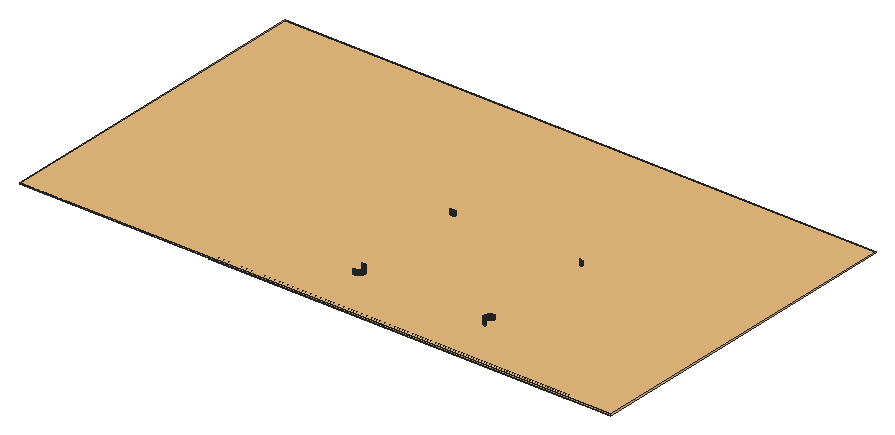
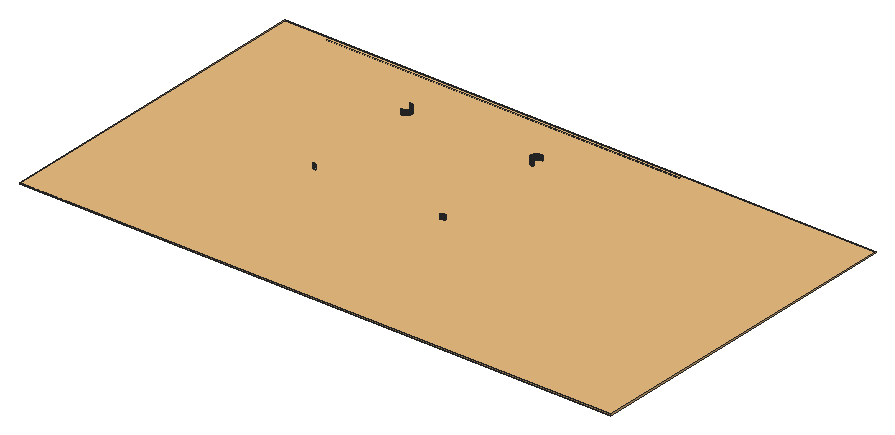
# SketchUp Ruby script. Lengths in inches.
U = 1.inch
M = Sketchup.active_model
def pt(a) = Geom::Point3d.new(a.map { |v| v * U })
def face(e, loops, mat)
  f = e.add_face(loops[0].map { |a| pt(a) })
  loops[1..].each { |l| e.add_face(l.map { |a| pt(a) }).erase! }
  f.material = f.back_material = mat if mat
  f
end
# faces: each face lists its corners as indices into pts; further lists are holes
def faces(e, pts, list, mat = nil) = list.each { |f| face(e, (f[0].is_a?(Array) ? f : [f]).map { |l| l.map { |i| pts[i] } }, mat) }
# xy, xz, yz: faces in a plane at the given z, y or x. An outline is a flat list of corners, or four numbers for a rectangle; further outlines are holes
def ring(l) = l.size == 4 ? [[l[0], l[1]], [l[2], l[1]], [l[2], l[3]], [l[0], l[3]]] : l.each_slice(2).to_a
def flat(e, list, mat, &to3) = list.each { |f| face(e, (f[0].is_a?(Array) ? f : [f]).map { |l| ring(l).map { |u, v| to3.(u, v) } }, mat) }
def xy(e, z, list, mat = nil) = flat(e, list, mat) { |x, y| [x, y, z] }
def xz(e, y, list, mat = nil) = flat(e, list, mat) { |x, z| [x, y, z] }
def yz(e, x, list, mat = nil) = flat(e, list, mat) { |y, z| [x, y, z] }
def lines(e, pts, list) = list.each { |a, b| e.add_line(pt(pts[a]), pt(pts[b])) }
# prism: a flat outline (further loops are holes) pulled along v
def prism(e, loops, v, mat = nil)
  f = face(e, loops, mat); d = Geom::Vector3d.new(v.map { |x| x * U })
  f.pushpull(f.normal.samedirection?(d) ? d.length : -d.length)
end
def box(e, o, s, mat = nil) = prism(e, [[o, [o[0] + s[0], o[1], o[2]], [o[0] + s[0], o[1] + s[1], o[2]], [o[0], o[1] + s[1], o[2]]]], [0, 0, s[2]], mat)
def at(x, y, z, deg = 0) = Geom::Transformation.translation(pt([x, y, z])) * Geom::Transformation.rotation(ORIGIN, Z_AXIS, deg.degrees)
def axes(o, x, y, z) = Geom::Transformation.new([*x, 0, *y, 0, *z, 0, *pt(o).to_a, 1])
def part(name) = M.definitions.add(name)
# library, detail: a bought-in or finely detailed component or shape, given as its bounding box
def library(name, o, s) = part(name).tap { |d| box(d.entities, o, s) }
def detail(e, o, s) = box(e.add_group.entities, o, s)
def put(e, d, t, mat = nil) = e.add_instance(d, t).tap { |i| i.material = mat if mat }
def group(e, t, mat = nil) = e.add_group.tap { |g| g.transformation = t; g.material = mat if mat }.entities
root = M.entities
M.materials.add("False Ceiling light").color = [253, 223, 143]
c1 = library("Group\#24",[0,0,-0.5],[314,176,0.5])
xz(root,159,[[133.5,107.5,323.38,108.5]])
xz(root,161,[[135.5,108,323.19,108.5]])
xz(root,185,[[189.84,108,189.92,111],[189.92,108,190,111],[190,108,190.08,111],[190.08,108,190.16,111],[259.34,108,259.42,111],
  [259.42,108,259.5,111],[259.5,108,259.58,111],[259.58,108,259.66,111]])
xz(root,191,[[189.84,108,189.92,111],[189.92,108,190,111],[190,108,190.08,111],[190.08,108,190.16,111],[259.34,108,259.42,111],
  [259.42,108,259.5,111],[259.5,108,259.58,111],[259.58,108,259.66,111]])
xz(root,249.5,[[189.84,108,189.92,111],[189.92,108,190,111],[190,108,190.08,111],[190.08,108,190.16,111],[259.34,108,259.42,111],
  [259.42,108,259.5,111],[259.5,108,259.58,111],[259.58,108,259.66,111]])
yz(root,193,[[187.84,108,187.92,111],[187.92,108,188,111],[188,108,188.08,111],[188.08,108,188.16,111]])
yz(root,256.5,[[187.84,108,187.92,111],[187.92,108,188,111],[188,108,188.08,111],[188.08,108,188.16,111]])
p = [[189.61,185.03,108],[189.53,185.04,108],[189.53,185.04,111],[189.61,185.03,111],[189.45,185.05,108],[189.45,185.05,111],
  [189.6875,185.02,108],[189.6875,185.02,111],[189.76,185.01,108],[189.76,185.01,111],[189.84,185,108],[189.84,185,111],
  [190.24,185.01,108],[190.16,185,108],[190.16,185,111],[190.24,185.01,111],[190.3125,185.02,108],[190.3125,185.02,111],
  [190.39,185.03,108],[190.39,185.03,111],[190.47,185.04,108],[190.47,185.04,111],[190.55,185.05,108],[190.55,185.05,111],
  [259.11,185.03,108],[259.03,185.04,108],[259.03,185.04,111],[259.11,185.03,111],[258.95,185.05,108],[258.95,185.05,111],
  [259.1875,185.02,108],[259.1875,185.02,111],[259.26,185.01,108],[259.26,185.01,111],[259.34,185,108],[259.34,185,111],
  [259.74,185.01,108],[259.66,185,108],[259.66,185,111],[259.74,185.01,111],[259.8125,185.02,108],[259.8125,185.02,111],
  [259.89,185.03,108],[259.89,185.03,111],[189.22,185.1,108],[189.15,185.125,108],[189.15,185.125,111],[189.22,185.1,111],
  [189.07,185.15,108],[189.07,185.15,111],[189.3,185.08,108],[189.3,185.08,111],[189.375,185.07,108],[189.375,185.07,111],
  [190.625,185.07,108],[190.625,185.07,111],[190.7,185.08,108],[190.7,185.08,111],[190.78,185.1,108],[190.78,185.1,111],
  [190.85,185.125,108],[190.85,185.125,111],[190.93,185.15,108],[190.93,185.15,111],[191,185.17,108],[191,185.17,111],
  [258.57,185.15,108],[258.5,185.17,108],[258.5,185.17,111],[258.57,185.15,111],[258.72,185.1,108],[258.65,185.125,108],
  [258.65,185.125,111],[258.72,185.1,111],[258.8,185.08,108],[258.8,185.08,111],[258.875,185.07,108],[258.875,185.07,111],
  [191.08,185.2,108],[191.08,185.2,111],[191.15,185.23,108],[191.15,185.23,111],[191.22,185.26,108],[191.22,185.26,111],
  [258.35,185.23,108],[258.28,185.26,108],[258.28,185.26,111],[258.35,185.23,111],[258.42,185.2,108],[258.42,185.2,111],
  [191.29,185.29,108],[191.29,185.29,111],[191.36,185.33,108],[191.36,185.33,111],[191.43,185.36,108],[191.43,185.36,111],
  [258.21,185.29,108],[258.14,185.33,108],[258.14,185.33,111],[258.21,185.29,111],[258.07,185.36,108],[258.07,185.36,111],
  [191.5,185.4,108],[191.5,185.4,111],[191.57,185.44,108],[191.57,185.44,111],[191.63,185.48,108],[191.63,185.48,111],
  [258,185.4,108],[257.93,185.44,108],[257.93,185.44,111],[258,185.4,111],[257.87,185.48,108],[257.87,185.48,111],
  [191.7,185.53,108],[191.7,185.53,111],[191.76,185.57,108],[191.76,185.57,111],[257.8,185.53,108],[257.74,185.57,108],
  [257.74,185.57,111],[257.8,185.53,111],[191.83,185.62,108],[191.83,185.62,111],[191.89,185.67,108],[191.89,185.67,111],
  [257.67,185.62,108],[257.61,185.67,108],[257.61,185.67,111],[257.67,185.62,111],[191.95,185.72,108],[191.95,185.72,111],
  [192.01,185.77,108],[192.01,185.77,111],[257.55,185.72,108],[257.49,185.77,108],[257.49,185.77,111],[257.55,185.72,111],
  [192.07,185.82,108],[192.07,185.82,111],[192.12,185.88,108],[192.12,185.88,111],[257.43,185.82,108],[257.43,185.82,111],
  [257.38,185.88,108],[257.38,185.88,111],[192.18,185.93,108],[192.18,185.93,111],[192.23,185.99,108],[192.23,185.99,111],
  [257.32,185.93,108],[257.32,185.93,111],[257.27,185.99,108],[257.27,185.99,111],[192.28,186.05,108],[192.28,186.05,111],
  [257.22,186.05,108],[257.22,186.05,111],[192.33,186.11,108],[192.33,186.11,111],[192.38,186.17,108],[192.38,186.17,111],
  [257.17,186.11,108],[257.12,186.17,108],[257.12,186.17,111],[257.17,186.11,111],[192.43,186.24,108],[192.43,186.24,111],
  [192.47,186.3,108],[192.47,186.3,111],[257.07,186.24,108],[257.03,186.3,108],[257.03,186.3,111],[257.07,186.24,111],
  [192.52,186.37,108],[192.52,186.37,111],[256.98,186.37,108],[256.98,186.37,111],[192.56,186.43,108],[192.56,186.43,111],
  [192.6,186.5,108],[192.6,186.5,111],[256.94,186.43,108],[256.94,186.43,111],[256.9,186.5,108],[256.9,186.5,111],
  [192.64,186.57,108],[192.64,186.57,111],[256.86,186.57,108],[256.86,186.57,111],[192.67,186.64,108],[192.67,186.64,111],
  [192.71,186.71,108],[192.71,186.71,111],[256.83,186.64,108],[256.83,186.64,111],[256.79,186.71,108],[256.79,186.71,111],
  [192.74,186.78,108],[192.74,186.78,111],[256.76,186.78,108],[256.76,186.78,111],[192.77,186.85,108],[192.77,186.85,111],
  [256.73,186.85,108],[256.73,186.85,111],[192.8,186.92,108],[192.8,186.92,111],[192.83,187,108],[192.83,187,111],
  [256.7,186.92,108],[256.7,186.92,111],[256.67,187,108],[256.67,187,111],[192.85,187.07,108],[192.85,187.07,111],
  [256.65,187.07,108],[256.65,187.07,111],[192.875,187.15,108],[192.875,187.15,111],[192.9,187.22,108],[192.9,187.22,111],
  [256.625,187.15,108],[256.625,187.15,111],[256.6,187.22,108],[256.6,187.22,111],[192.92,187.3,108],[192.92,187.3,111],
  [256.58,187.3,108],[256.58,187.3,111],[192.93,187.375,108],[192.93,187.375,111],[256.57,187.375,108],[256.57,187.375,111],
  [192.95,187.45,108],[192.95,187.45,111],[256.55,187.45,108],[256.55,187.45,111],[192.96,187.53,108],[192.96,187.53,111],
  [192.97,187.61,108],[192.97,187.61,111],[256.54,187.53,108],[256.54,187.53,111],[256.53,187.61,108],[256.53,187.61,111],
  [192.98,187.6875,108],[192.98,187.6875,111],[256.52,187.6875,108],[256.52,187.6875,111],[192.99,187.76,108],[192.99,187.76,111],
  [256.51,187.76,108],[256.51,187.76,111],[193,187.84,108],[193,187.84,111],[256.5,187.84,108],[256.5,187.84,111],
  [192.99,188.24,108],[193,188.16,108],[193,188.16,111],[192.99,188.24,111],[192.98,188.3125,108],[192.98,188.3125,111],
  [256.5,188.16,108],[256.51,188.24,108],[256.51,188.24,111],[256.5,188.16,111],[256.52,188.3125,108],[256.52,188.3125,111],
  [192.97,188.39,108],[192.97,188.39,111],[256.53,188.39,108],[256.53,188.39,111],[192.96,188.47,108],[192.96,188.47,111],
  [256.54,188.47,108],[256.54,188.47,111],[192.95,188.55,108],[192.95,188.55,111],[192.93,188.625,108],[192.93,188.625,111],
  [256.55,188.55,108],[256.55,188.55,111],[256.57,188.625,108],[256.57,188.625,111],[192.92,188.7,108],[192.92,188.7,111],
  [256.58,188.7,108],[256.58,188.7,111],[192.9,188.78,108],[192.9,188.78,111],[256.6,188.78,108],[256.6,188.78,111],
  [192.875,188.85,108],[192.875,188.85,111],[256.625,188.85,108],[256.625,188.85,111],[192.83,189,108],[192.85,188.93,108],
  [192.85,188.93,111],[192.83,189,111],[256.65,188.93,108],[256.65,188.93,111],[256.67,189,108],[256.67,189,111],
  [192.8,189.08,108],[192.8,189.08,111],[256.7,189.08,108],[256.7,189.08,111],[192.74,189.22,108],[192.77,189.15,108],
  [192.77,189.15,111],[192.74,189.22,111],[256.73,189.15,108],[256.73,189.15,111],[256.76,189.22,108],[256.76,189.22,111],
  [192.71,189.29,108],[192.71,189.29,111],[256.79,189.29,108],[256.79,189.29,111],[192.67,189.36,108],[192.67,189.36,111],
  [256.83,189.36,108],[256.83,189.36,111],[192.64,189.43,108],[192.64,189.43,111],[192.6,189.5,108],[192.6,189.5,111],
  [256.86,189.43,108],[256.86,189.43,111],[256.9,189.5,108],[256.9,189.5,111],[192.56,189.57,108],[192.56,189.57,111],
  [256.94,189.57,108],[256.94,189.57,111],[192.52,189.63,108],[192.52,189.63,111],[192.47,189.7,108],[192.47,189.7,111],
  [256.98,189.63,108],[256.98,189.63,111],[257.03,189.7,108],[257.03,189.7,111],[192.43,189.76,108],[192.43,189.76,111],
  [257.07,189.76,108],[257.07,189.76,111],[192.33,189.89,108],[192.38,189.83,108],[192.38,189.83,111],[192.33,189.89,111],
  [257.12,189.83,108],[257.12,189.83,111],[257.17,189.89,108],[257.17,189.89,111],[192.23,190.01,108],[192.28,189.95,108],
  [192.28,189.95,111],[192.23,190.01,111],[257.22,189.95,108],[257.22,189.95,111],[257.27,190.01,108],[257.27,190.01,111],
  [192.18,190.07,108],[192.18,190.07,111],[257.32,190.07,108],[257.32,190.07,111],[192.12,190.12,108],[192.12,190.12,111],
  [192.07,190.18,108],[192.07,190.18,111],[257.38,190.12,108],[257.38,190.12,111],[257.43,190.18,108],[257.43,190.18,111],
  [191.95,190.28,108],[192.01,190.23,108],[192.01,190.23,111],[191.95,190.28,111],[257.49,190.23,108],[257.49,190.23,111],
  [257.55,190.28,108],[257.55,190.28,111],[191.83,190.38,108],[191.89,190.33,108],[191.89,190.33,111],[191.83,190.38,111],
  [257.61,190.33,108],[257.61,190.33,111],[257.67,190.38,108],[257.67,190.38,111],[191.7,190.47,108],[191.76,190.43,108],
  [191.76,190.43,111],[191.7,190.47,111],[257.74,190.43,108],[257.74,190.43,111],[257.8,190.47,108],[257.8,190.47,111],
  [191.63,190.52,108],[191.63,190.52,111],[191.57,190.56,108],[191.57,190.56,111],[257.87,190.52,108],[257.87,190.52,111],
  [257.93,190.56,108],[257.93,190.56,111],[191.43,190.64,108],[191.5,190.6,108],[191.5,190.6,111],[191.43,190.64,111],
  [191.36,190.67,108],[191.36,190.67,111],[258,190.6,108],[258,190.6,111],[258.07,190.64,108],[258.07,190.64,111],
  [258.14,190.67,108],[258.14,190.67,111],[191.15,190.77,108],[191.22,190.74,108],[191.22,190.74,111],[191.15,190.77,111],
  [191.29,190.71,108],[191.29,190.71,111],[258.21,190.71,108],[258.21,190.71,111],[258.28,190.74,108],[258.28,190.74,111],
  [258.35,190.77,108],[258.35,190.77,111],[190.93,190.85,108],[191,190.83,108],[191,190.83,111],[190.93,190.85,111],
  [191.08,190.8,108],[191.08,190.8,111],[258.42,190.8,108],[258.42,190.8,111],[258.5,190.83,108],[258.5,190.83,111],
  [258.57,190.85,108],[258.57,190.85,111],[189.07,190.85,108],[189.15,190.875,108],[189.15,190.875,111],[189.07,190.85,111],
  [189.22,190.9,108],[189.22,190.9,111],[189.3,190.92,108],[189.3,190.92,111],[189.375,190.93,108],[189.375,190.93,111],
  [189.45,190.95,108],[189.45,190.95,111],[189.53,190.96,108],[189.53,190.96,111],[190.55,190.95,108],[190.625,190.93,108],
  [190.625,190.93,111],[190.55,190.95,111],[190.47,190.96,108],[190.47,190.96,111],[190.7,190.92,108],[190.7,190.92,111],
  [190.78,190.9,108],[190.78,190.9,111],[190.85,190.875,108],[190.85,190.875,111],[258.65,190.875,108],[258.65,190.875,111],
  [258.72,190.9,108],[258.72,190.9,111],[258.8,190.92,108],[258.8,190.92,111],[258.875,190.93,108],[258.875,190.93,111],
  [258.95,190.95,108],[258.95,190.95,111],[259.03,190.96,108],[259.03,190.96,111],[189.61,190.97,108],[189.61,190.97,111],
  [189.6875,190.98,108],[189.6875,190.98,111],[189.76,190.99,108],[189.76,190.99,111],[189.84,191,108],[189.84,191,111],
  [190.24,190.99,108],[190.3125,190.98,108],[190.3125,190.98,111],[190.24,190.99,111],[190.16,191,108],[190.16,191,111],
  [190.39,190.97,108],[190.39,190.97,111],[259.11,190.97,108],[259.11,190.97,111],[259.1875,190.98,108],[259.1875,190.98,111],
  [259.26,190.99,108],[259.26,190.99,111],[259.34,191,108],[259.34,191,111],[259.74,190.99,108],[259.8125,190.98,108],
  [259.8125,190.98,111],[259.74,190.99,111],[259.66,191,108],[259.66,191,111],[259.89,190.97,108],[259.89,190.97,111],
  [259.97,190.96,108],[259.97,190.96,111],[189.61,249.53,108],[189.53,249.54,108],[189.53,249.54,111],[189.61,249.53,111],
  [189.45,249.55,108],[189.45,249.55,111],[189.6875,249.52,108],[189.6875,249.52,111],[189.76,249.51,108],[189.76,249.51,111],
  [189.84,249.5,108],[189.84,249.5,111],[190.24,249.51,108],[190.16,249.5,108],[190.16,249.5,111],[190.24,249.51,111],
  [190.3125,249.52,108],[190.3125,249.52,111],[190.39,249.53,108],[190.39,249.53,111],[190.47,249.54,108],[190.47,249.54,111],
  [190.55,249.55,108],[190.55,249.55,111],[259.11,249.53,108],[259.03,249.54,108],[259.03,249.54,111],[259.11,249.53,111],
  [258.95,249.55,108],[258.95,249.55,111],[259.1875,249.52,108],[259.1875,249.52,111],[259.26,249.51,108],[259.26,249.51,111],
  [259.34,249.5,108],[259.34,249.5,111],[259.74,249.51,108],[259.66,249.5,108],[259.66,249.5,111],[259.74,249.51,111],
  [259.8125,249.52,108],[259.8125,249.52,111],[259.89,249.53,108],[259.89,249.53,111],[189.22,249.6,108],[189.15,249.625,108],
  [189.15,249.625,111],[189.22,249.6,111],[189.07,249.65,108],[189.07,249.65,111],[189.3,249.58,108],[189.3,249.58,111],
  [189.375,249.57,108],[189.375,249.57,111],[190.625,249.57,108],[190.625,249.57,111],[190.7,249.58,108],[190.7,249.58,111],
  [190.78,249.6,108],[190.78,249.6,111],[190.85,249.625,108],[190.85,249.625,111],[190.93,249.65,108],[190.93,249.65,111],
  [191,249.67,108],[191,249.67,111],[258.57,249.65,108],[258.5,249.67,108],[258.5,249.67,111],[258.57,249.65,111],
  [258.72,249.6,108],[258.65,249.625,108],[258.65,249.625,111],[258.72,249.6,111],[258.8,249.58,108],[258.8,249.58,111],
  [258.875,249.57,108],[258.875,249.57,111],[191.08,249.7,108],[191.08,249.7,111],[191.15,249.73,108],[191.15,249.73,111],
  [191.22,249.76,108],[191.22,249.76,111],[258.35,249.73,108],[258.28,249.76,108],[258.28,249.76,111],[258.35,249.73,111],
  [258.42,249.7,108],[258.42,249.7,111],[191.29,249.79,108],[191.29,249.79,111],[191.36,249.83,108],[191.36,249.83,111],
  [191.43,249.86,108],[191.43,249.86,111],[258.21,249.79,108],[258.14,249.83,108],[258.14,249.83,111],[258.21,249.79,111],
  [258.07,249.86,108],[258.07,249.86,111],[191.5,249.9,108],[191.5,249.9,111],[191.57,249.94,108],[191.57,249.94,111],
  [191.63,249.98,108],[191.63,249.98,111],[258,249.9,108],[257.93,249.94,108],[257.93,249.94,111],[258,249.9,111],
  [257.87,249.98,108],[257.87,249.98,111],[191.7,250.03,108],[191.7,250.03,111],[257.8,250.03,108],[257.74,250.07,108],
  [257.74,250.07,111],[257.8,250.03,111]]
faces(root,p,[[0,1,2,3],[1,4,5,2],[6,0,3,7],[8,6,7,9],[10,8,9,11],[12,13,14,15],[16,12,15,17],[18,16,17,19],
  [20,18,19,21],[22,20,21,23],[24,25,26,27],[25,28,29,26],[30,24,27,31],[32,30,31,33],[34,32,33,35],[36,37,38,39],
  [40,36,39,41],[42,40,41,43],[44,45,46,47],[45,48,49,46],[50,44,47,51],[52,50,51,53],[4,52,53,5],[54,22,23,55],
  [56,54,55,57],[58,56,57,59],[60,58,59,61],[62,60,61,63],[64,62,63,65],[66,67,68,69],[70,71,72,73],[71,66,69,72],
  [74,70,73,75],[76,74,75,77],[28,76,77,29],[78,64,65,79],[80,78,79,81],[82,80,81,83],[84,85,86,87],[67,88,89,68],
  [88,84,87,89],[90,82,83,91],[92,90,91,93],[94,92,93,95],[96,97,98,99],[97,100,101,98],[85,96,99,86],[102,94,95,103],
  [104,102,103,105],[106,104,105,107],[108,109,110,111],[109,112,113,110],[100,108,111,101],[114,106,107,115],[116,114,115,117],[118,119,120,121],
  [112,118,121,113],[122,116,117,123],[124,122,123,125],[126,127,128,129],[119,126,129,120],[130,124,125,131],[132,130,131,133],[134,135,136,137],
  [127,134,137,128],[138,132,133,139],[140,138,139,141],[135,142,143,136],[142,144,145,143],[146,140,141,147],[148,146,147,149],[144,150,151,145],
  [150,152,153,151],[154,148,149,155],[152,156,157,153],[158,154,155,159],[160,158,159,161],[162,163,164,165],[156,162,165,157],[166,160,161,167],
  [168,166,167,169],[170,171,172,173],[163,170,173,164],[174,168,169,175],[171,176,177,172],[178,174,175,179],[180,178,179,181],[176,182,183,177],
  [182,184,185,183],[186,180,181,187],[184,188,189,185],[190,186,187,191],[192,190,191,193],[188,194,195,189],[194,196,197,195],[198,192,193,199],
  [196,200,201,197],[202,198,199,203],[200,204,205,201],[206,202,203,207],[208,206,207,209],[204,210,211,205],[210,212,213,211],[214,208,209,215],
  [212,216,217,213],[218,214,215,219],[220,218,219,221],[216,222,223,217],[222,224,225,223],[226,220,221,227],[224,228,229,225],[230,226,227,231],
  [228,232,233,229],[234,230,231,235],[232,236,237,233],[238,234,235,239],[240,238,239,241],[236,242,243,237],[242,244,245,243],[246,240,241,247],
  [244,248,249,245],[250,246,247,251],[248,252,253,249],[254,250,251,255],[252,256,257,253],[258,259,260,261],[262,258,261,263],[264,265,266,267],
  [265,268,269,266],[270,262,263,271],[268,272,273,269],[274,270,271,275],[272,276,277,273],[278,274,275,279],[280,278,279,281],[276,282,283,277],
  [282,284,285,283],[286,280,281,287],[284,288,289,285],[290,286,287,291],[288,292,293,289],[294,290,291,295],[292,296,297,293],[298,299,300,301],
  [299,294,295,300],[296,302,303,297],[302,304,305,303],[306,298,301,307],[304,308,309,305],[310,311,312,313],[311,306,307,312],[308,314,315,309],
  [314,316,317,315],[318,310,313,319],[316,320,321,317],[322,318,319,323],[320,324,325,321],[326,322,323,327],[328,326,327,329],[324,330,331,325],
  [330,332,333,331],[334,328,329,335],[332,336,337,333],[338,334,335,339],[340,338,339,341],[336,342,343,337],[342,344,345,343],[346,340,341,347],
  [344,348,349,345],[350,351,352,353],[351,346,347,352],[348,354,355,349],[354,356,357,355],[358,359,360,361],[359,350,353,360],[356,362,363,357],
  [362,364,365,363],[366,358,361,367],[364,368,369,365],[370,366,367,371],[372,370,371,373],[368,374,375,369],[374,376,377,375],[378,379,380,381],
  [379,372,373,380],[376,382,383,377],[382,384,385,383],[386,387,388,389],[387,378,381,388],[384,390,391,385],[390,392,393,391],[394,395,396,397],
  [395,386,389,396],[392,398,399,393],[398,400,401,399],[402,394,397,403],[404,402,403,405],[400,406,407,401],[406,408,409,407],[410,411,412,413],
  [414,410,413,415],[411,404,405,412],[408,416,417,409],[416,418,419,417],[418,420,421,419],[422,423,424,425],[423,426,427,424],[426,414,415,427],
  [420,428,429,421],[428,430,431,429],[430,432,433,431],[434,435,436,437],[435,438,439,436],[438,422,425,439],[432,440,441,433],[440,442,443,441],
  [442,444,445,443],[446,447,448,449],[447,450,451,448],[450,452,453,451],[452,454,455,453],[454,456,457,455],[456,458,459,457],[460,461,462,463],
  [464,460,463,465],[461,466,467,462],[466,468,469,467],[468,470,471,469],[470,434,437,471],[444,472,473,445],[472,474,475,473],[474,476,477,475],
  [476,478,479,477],[478,480,481,479],[480,482,483,481],[458,484,485,459],[484,486,487,485],[486,488,489,487],[488,490,491,489],[492,493,494,495],
  [496,492,495,497],[493,498,499,494],[498,464,465,499],[482,500,501,483],[500,502,503,501],[502,504,505,503],[504,506,507,505],[508,509,510,511],
  [512,508,511,513],[509,514,515,510],[514,516,517,515],[518,519,520,521],[519,522,523,520],[524,518,521,525],[526,524,525,527],[528,526,527,529],
  [530,531,532,533],[534,530,533,535],[536,534,535,537],[538,536,537,539],[540,538,539,541],[542,543,544,545],[543,546,547,544],[548,542,545,549],
  [550,548,549,551],[552,550,551,553],[554,555,556,557],[558,554,557,559],[560,558,559,561],[562,563,564,565],[563,566,567,564],[568,562,565,569],
  [570,568,569,571],[522,570,571,523],[572,540,541,573],[574,572,573,575],[576,574,575,577],[578,576,577,579],[580,578,579,581],[582,580,581,583],
  [584,585,586,587],[588,589,590,591],[589,584,587,590],[592,588,591,593],[594,592,593,595],[546,594,595,547],[596,582,583,597],[598,596,597,599],
  [600,598,599,601],[602,603,604,605],[585,606,607,586],[606,602,605,607],[608,600,601,609],[610,608,609,611],[612,610,611,613],[614,615,616,617],
  [615,618,619,616],[603,614,617,604],[620,612,613,621],[622,620,621,623],[624,622,623,625],[626,627,628,629],[627,630,631,628],[618,626,629,619],
  [632,624,625,633],[634,635,636,637],[630,634,637,631]])
put(root,c1,at(33,159,108.5),"False Ceiling light")
